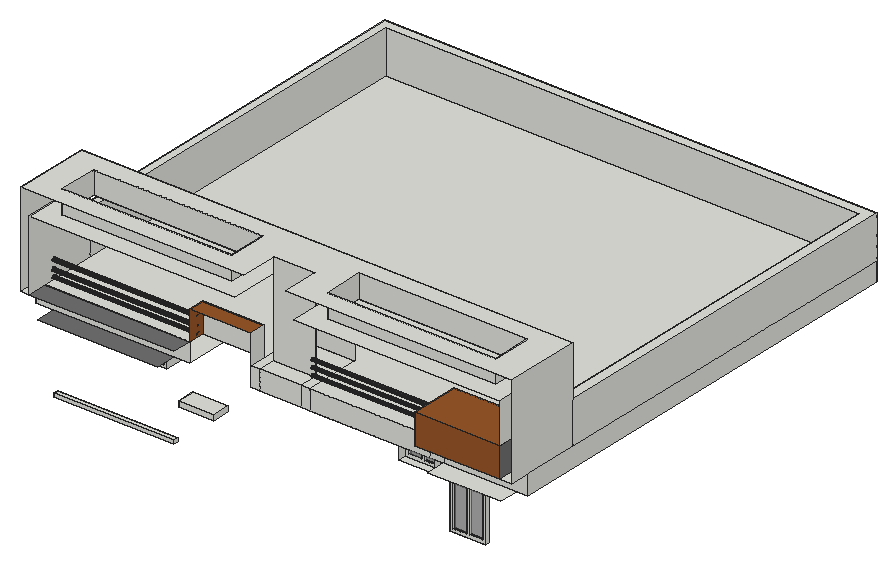
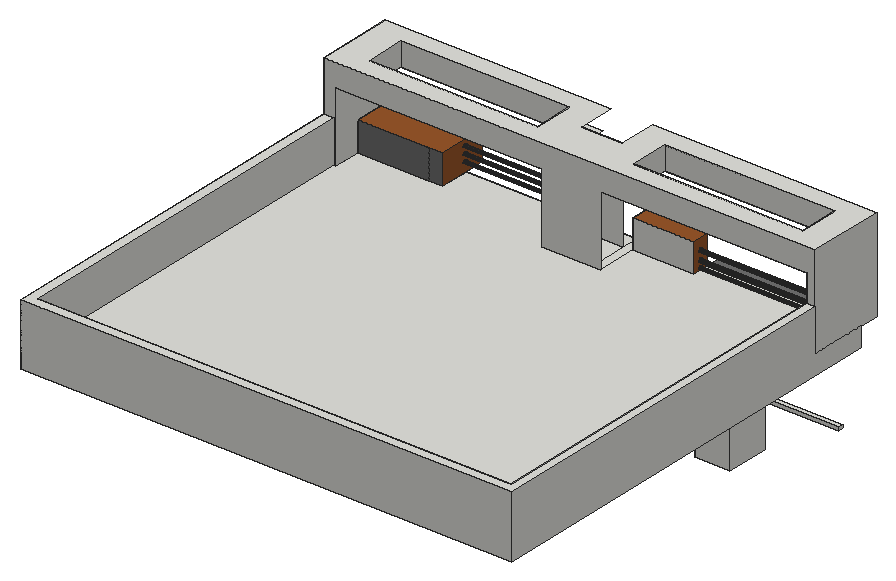
# SketchUp Ruby script. Lengths in inches.
U = 1.inch
M = Sketchup.active_model
def pt(a) = Geom::Point3d.new(a.map { |v| v * U })
def face(e, loops, mat)
  f = e.add_face(loops[0].map { |a| pt(a) })
  loops[1..].each { |l| e.add_face(l.map { |a| pt(a) }).erase! }
  f.material = f.back_material = mat if mat
  f
end
# faces: each face lists its corners as indices into pts; further lists are holes
def faces(e, pts, list, mat = nil) = list.each { |f| face(e, (f[0].is_a?(Array) ? f : [f]).map { |l| l.map { |i| pts[i] } }, mat) }
# xy, xz, yz: faces in a plane at the given z, y or x. An outline is a flat list of corners, or four numbers for a rectangle; further outlines are holes
def ring(l) = l.size == 4 ? [[l[0], l[1]], [l[2], l[1]], [l[2], l[3]], [l[0], l[3]]] : l.each_slice(2).to_a
def flat(e, list, mat, &to3) = list.each { |f| face(e, (f[0].is_a?(Array) ? f : [f]).map { |l| ring(l).map { |u, v| to3.(u, v) } }, mat) }
def xy(e, z, list, mat = nil) = flat(e, list, mat) { |x, y| [x, y, z] }
def xz(e, y, list, mat = nil) = flat(e, list, mat) { |x, z| [x, y, z] }
def yz(e, x, list, mat = nil) = flat(e, list, mat) { |y, z| [x, y, z] }
def lines(e, pts, list) = list.each { |a, b| e.add_line(pt(pts[a]), pt(pts[b])) }
# prism: a flat outline (further loops are holes) pulled along v
def prism(e, loops, v, mat = nil)
  f = face(e, loops, mat); d = Geom::Vector3d.new(v.map { |x| x * U })
  f.pushpull(f.normal.samedirection?(d) ? d.length : -d.length)
end
def box(e, o, s, mat = nil) = prism(e, [[o, [o[0] + s[0], o[1], o[2]], [o[0] + s[0], o[1] + s[1], o[2]], [o[0], o[1] + s[1], o[2]]]], [0, 0, s[2]], mat)
def at(x, y, z, deg = 0) = Geom::Transformation.translation(pt([x, y, z])) * Geom::Transformation.rotation(ORIGIN, Z_AXIS, deg.degrees)
def axes(o, x, y, z) = Geom::Transformation.new([*x, 0, *y, 0, *z, 0, *pt(o).to_a, 1])
def part(name) = M.definitions.add(name)
# library, detail: a bought-in or finely detailed component or shape, given as its bounding box
def library(name, o, s) = part(name).tap { |d| box(d.entities, o, s) }
def detail(e, o, s) = box(e.add_group.entities, o, s)
def put(e, d, t, mat = nil) = e.add_instance(d, t).tap { |i| i.material = mat if mat }
def group(e, t, mat = nil) = e.add_group.tap { |g| g.transformation = t; g.material = mat if mat }.entities
root = M.entities
M.materials.add("Generic").color = [112, 112, 112]
M.materials.add("[Color M07]").color = [58, 58, 58]
M.materials.add("[Translucent Glass Gray]").color = [128, 128, 128]
M.materials["[Translucent Glass Gray]"].alpha = 0.5
M.materials.add("[Wood Cherry Original]").color = [152, 86, 42]
c1 = part("Group\#2")
xy(c1.entities,0,[[0,0,49,5]])
xy(c1.entities,4.23,[[4.23,0,22.39,2],[26.61,0,44.77,2]])
xy(c1.entities,60.71,[[4.23,0,22.39,2],[26.61,0,44.77,2]])
xy(c1.entities,64.9375,[[0,0,49,5]])
xz(c1.entities,0,[[[0,0,49,64.9375],[26.61,4.23,44.77,60.71],[4.23,4.23,22.39,60.71]]])
xz(c1.entities,2,[[4.23,4.23,22.39,60.71],[26.61,4.23,44.77,60.71]],"[Translucent Glass Gray]")
xz(c1.entities,5,[[0,0,49,64.9375]],"[Translucent Glass Gray]")
yz(c1.entities,0,[[0,0,5,64.9375]])
yz(c1.entities,4.23,[[0,4.23,2,60.71]])
yz(c1.entities,22.39,[[0,4.23,2,60.71]])
yz(c1.entities,26.61,[[0,4.23,2,60.71]])
yz(c1.entities,44.77,[[0,4.23,2,60.71]])
yz(c1.entities,49,[[0,0,5,64.9375]])
box(root,[24,106.875,891],[165.05,7.3125,4.75])
xy(root,903.58,[[46.11,213.8125,95.11,273.4375],[414.49,213.8125,463.49,273.4375]])
xy(root,957.51,[[216.02,81.875,264.46,106.875]])
xy(root,964.95,[[216.02,81.875,264.46,106.875]])
xy(root,968.52,[[46.11,213.8125,95.11,273.4375],[414.49,213.8125,463.49,273.4375]])
xy(root,973,[[124.42,213.8125,178.54,273.4375],[492.79,213.8125,546.92,273.4375]])
xy(root,998.375,[[561.52,79.8125,661.8125,106.875],[24,106.875,211.17,213.8125],[295.66,106.875,295.66,249.5625,347.59,249.5625,347.59,151,307.66,151,307.66,106.875],[307.66,106.875,364.97,151],[364.97,106.875,364.97,151,347.59,151,347.59,249.5625,376.97,249.5625,376.97,106.875],
  [376.97,106.875,561.52,213.8125]])
xy(root,998.375,[[24,79.8125,189.05,106.875]],"Generic")
xy(root,1025.25,[[0,79.8125,12,106.875],[659.375,79.8125,676.6875,106.875],[0,106.875,12,184.9375],[12,106.875,211.17,106.875,211.17,129.125,295.66,129.125,295.66,184.9375,376.97,184.9375,376.97,106.875,542.64,106.875,542.64,147.5,659.375,147.5,659.375,184.9375,662.75,184.9375,662.75,693.375,12,693.375],[295.66,106.875,307.66,184.9375],
  [307.66,106.875,364.97,130.875],[364.97,106.875,376.97,106.875,376.97,184.9375,307.66,184.9375,307.66,130.875,364.97,130.875],[659.375,106.875,676.6875,184.9375]])
xy(root,1025.25,[[12,79.8125,211.17,106.875],[542.64,79.8125,659.375,106.875],[542.64,106.875,561.52,147.5],[561.52,106.875,659.375,147.5]],"Generic")
xy(root,1065.0625,[[211.17,106.875,295.66,129.125]],"[Wood Cherry Original]")
xy(root,1066.4375,[[542.64,79.8125,659.375,147.5]],"[Wood Cherry Original]")
xy(root,1084,[[0,184.9375,12,184.9375,12,693.375,662.75,693.375,662.75,184.9375,676.6875,184.9375,676.6875,706.875,0,706.875]])
xy(root,1121.625,[[[12,79.8125,295.66,184.9375],[37.42,105.23,270.24,159.52]],[[376.97,79.8125,659.375,184.9375],[402.39,105.23,633.96,159.52]]])
xy(root,1153.3125,[[[0,79.8125,307.66,79.8125,307.66,130.875,364.97,130.875,364.97,79.8125,676.6875,79.8125,676.6875,184.9375,0,184.9375],[37.42,105.23,270.24,159.52],[402.39,105.23,633.96,159.52]]])
xz(root,79.8125,[[542.64,1025.25,659.375,1066.4375]],"[Wood Cherry Original]")
xz(root,81.875,[[216.02,957.51,264.46,964.95]])
xz(root,105.23,[[37.42,1121.625,270.24,1153.3125],[402.39,1121.625,633.96,1153.3125]])
xz(root,106.875,[[0,998.375,211.17,1025.25],[295.66,998.375,307.66,1025.25],[307.66,998.375,364.97,1025.25],[364.97,998.375,376.97,1025.25],[376.97,998.375,542.64,1025.25],
  [542.64,998.375,561.52,1025.25],[561.52,998.375,676.6875,1025.25]])
xz(root,129.125,[[211.17,1025.25,295.66,1065.0625]])
xz(root,130.875,[[307.66,1025.25,364.97,1153.3125]])
xz(root,147.5,[[542.64,1025.25,561.52,1066.4375],[561.52,1025.25,659.375,1066.4375]],"Generic")
xz(root,159.52,[[37.42,1121.625,270.24,1153.3125],[402.39,1121.625,633.96,1153.3125]])
xz(root,184.9375,[[0,1025.25,12,1084],[295.66,1025.25,295.66,1121.625,12,1121.625,12,1084,0,1084,0,1153.3125,676.6875,1153.3125,676.6875,1084,662.75,1084,662.75,1071.0625,659.375,1071.0625,659.375,1121.625,376.97,1121.625,376.97,1025.25],[659.375,1025.25,662.75,1071.0625],[662.75,1025.25,676.6875,1084]])
xz(root,273.4375,[[46.11,903.58,95.11,968.52],[414.49,903.58,463.49,968.52]])
xz(root,693.375,[[12,1025.25,662.75,1084]])
xz(root,706.875,[[0,998.375,676.6875,1084]])
yz(root,0,[[106.875,998.375,106.875,1025.25,184.9375,1025.25,184.9375,1084,706.875,1084,706.875,998.375],[79.8125,1025.25,184.9375,1153.3125]])
yz(root,12,[[[79.8125,1025.25,184.9375,1121.625],[120.64,1049.14,120.125,1049.16,119.625,1049.31,119.18,1049.59,118.82,1049.97,118.58,1050.43,118.46,1050.94,118.48,1051.46,118.63,1051.96,118.9,1052.4,119.28,1052.76,119.75,1053,120.25,1053.12,120.78,1053.1,121.28,1052.95,121.72,1052.68,122.08,1052.3,122.32,1051.83,122.44,1051.33,122.42,1050.8,122.27,1050.3,122,1049.86,121.61,1049.5,121.15,1049.26],[120.45,1036.69,119.93,1036.76,119.45,1036.96,119.04,1037.28,118.72,1037.69,118.52,1038.18,118.45,1038.69,118.52,1039.21,118.72,1039.69,119.04,1040.11,119.45,1040.43,119.93,1040.625,120.45,1040.69,120.97,1040.625,121.45,1040.43,121.86,1040.11,122.18,1039.69,122.38,1039.21,122.45,1038.69,122.38,1038.18,122.18,1037.69,121.86,1037.28,121.45,1036.96,120.97,1036.76],[120.45,1027.44,119.93,1027.51,119.45,1027.71,119.04,1028.03,118.72,1028.44,118.52,1028.93,118.45,1029.44,118.52,1029.96,118.72,1030.44,119.04,1030.86,119.45,1031.18,119.93,1031.375,120.45,1031.44,120.97,1031.375,121.45,1031.18,121.86,1030.86,122.18,1030.44,122.38,1029.96,122.45,1029.44,122.38,1028.93,122.18,1028.44,121.86,1028.03,121.45,1027.71,120.97,1027.51]],[184.9375,1025.25,693.375,1084]])
yz(root,37.42,[[105.23,1121.625,159.52,1153.3125]])
yz(root,46.11,[[213.8125,903.58,273.4375,968.52]])
yz(root,95.11,[[213.8125,903.58,273.4375,968.52]])
yz(root,211.17,[[[106.875,1025.25,129.125,1065.0625],[120.64,1049.14,121.15,1049.26,121.61,1049.5,122,1049.86,122.27,1050.3,122.42,1050.8,122.44,1051.33,122.32,1051.83,122.08,1052.3,121.72,1052.68,121.28,1052.95,120.78,1053.1,120.25,1053.12,119.75,1053,119.28,1052.76,118.9,1052.4,118.63,1051.96,118.48,1051.46,118.46,1050.94,118.58,1050.43,118.82,1049.97,119.18,1049.59,119.625,1049.31,120.125,1049.16],[120.45,1027.44,120.97,1027.51,121.45,1027.71,121.86,1028.03,122.18,1028.44,122.38,1028.93,122.45,1029.44,122.38,1029.96,122.18,1030.44,121.86,1030.86,121.45,1031.18,120.97,1031.375,120.45,1031.44,119.93,1031.375,119.45,1031.18,119.04,1030.86,118.72,1030.44,118.52,1029.96,118.45,1029.44,118.52,1028.93,118.72,1028.44,119.04,1028.03,119.45,1027.71,119.93,1027.51],[120.45,1036.69,120.97,1036.76,121.45,1036.96,121.86,1037.28,122.18,1037.69,122.38,1038.18,122.45,1038.69,122.38,1039.21,122.18,1039.69,121.86,1040.11,121.45,1040.43,120.97,1040.625,120.45,1040.69,119.93,1040.625,119.45,1040.43,119.04,1040.11,118.72,1039.69,118.52,1039.21,118.45,1038.69,118.52,1038.18,118.72,1037.69,119.04,1037.28,119.45,1036.96,119.93,1036.76]],[120.45,1027.44,120.97,1027.51,121.45,1027.71,121.86,1028.03,122.18,1028.44,122.38,1028.93,122.45,1029.44,122.38,1029.96,122.18,1030.44,121.86,1030.86,121.45,1031.18,120.97,1031.375,120.45,1031.44,119.93,1031.375,119.45,1031.18,119.04,1030.86,118.72,1030.44,118.52,1029.96,118.45,1029.44,118.52,1028.93,118.72,1028.44,119.04,1028.03,119.45,1027.71,119.93,1027.51],[120.45,1036.69,120.97,1036.76,121.45,1036.96,121.86,1037.28,122.18,1037.69,122.38,1038.18,122.45,1038.69,122.38,1039.21,122.18,1039.69,121.86,1040.11,121.45,1040.43,120.97,1040.625,120.45,1040.69,119.93,1040.625,119.45,1040.43,119.04,1040.11,118.72,1039.69,118.52,1039.21,118.45,1038.69,118.52,1038.18,118.72,1037.69,119.04,1037.28,119.45,1036.96,119.93,1036.76],[120.64,1049.14,121.15,1049.26,121.61,1049.5,122,1049.86,122.27,1050.3,122.42,1050.8,122.44,1051.33,122.32,1051.83,122.08,1052.3,121.72,1052.68,121.28,1052.95,120.78,1053.1,120.25,1053.12,119.75,1053,119.28,1052.76,118.9,1052.4,118.63,1051.96,118.48,1051.46,118.46,1050.94,118.58,1050.43,118.82,1049.97,119.18,1049.59,119.625,1049.31,120.125,1049.16]],"[Wood Cherry Original]")
yz(root,216.02,[[81.875,957.51,106.875,964.95]])
yz(root,264.46,[[81.875,957.51,106.875,964.95]])
yz(root,270.24,[[105.23,1121.625,159.52,1153.3125]])
yz(root,295.66,[[106.875,1025.25,129.125,1065.0625]])
yz(root,402.39,[[105.23,1121.625,159.52,1153.3125]])
yz(root,414.49,[[213.8125,903.58,273.4375,968.52]])
yz(root,463.49,[[213.8125,903.58,273.4375,968.52]])
yz(root,542.64,[[[79.8125,1025.25,147.5,1066.4375],[111.28,1047.72,111.79,1047.78,112.28,1047.98,112.69,1048.3,113.01,1048.72,113.21,1049.2,113.28,1049.72,113.21,1050.23,113.01,1050.72,112.69,1051.13,112.28,1051.45,111.79,1051.65,111.28,1051.72,110.76,1051.65,110.28,1051.45,109.86,1051.13,109.55,1050.72,109.35,1050.23,109.28,1049.72,109.35,1049.2,109.55,1048.72,109.86,1048.3,110.28,1047.98,110.76,1047.78],[111.28,1038.03,111.79,1038.1,112.28,1038.3,112.69,1038.61,113.01,1039.03,113.21,1039.51,113.28,1040.03,113.21,1040.55,113.01,1041.03,112.69,1041.44,112.28,1041.76,111.79,1041.96,111.28,1042.03,110.76,1041.96,110.28,1041.76,109.86,1041.44,109.55,1041.03,109.35,1040.55,109.28,1040.03,109.35,1039.51,109.55,1039.03,109.86,1038.61,110.28,1038.3,110.76,1038.1],[111.28,1057.4,111.79,1057.47,112.28,1057.67,112.69,1057.99,113.01,1058.4,113.21,1058.89,113.28,1059.4,113.21,1059.92,113.01,1060.4,112.69,1060.82,112.28,1061.14,111.79,1061.34,111.28,1061.4,110.76,1061.34,110.28,1061.14,109.86,1060.82,109.55,1060.4,109.35,1059.92,109.28,1059.4,109.35,1058.89,109.55,1058.4,109.86,1057.99,110.28,1057.67,110.76,1057.47]],[111.28,1038.03,111.79,1038.1,112.28,1038.3,112.69,1038.61,113.01,1039.03,113.21,1039.51,113.28,1040.03,113.21,1040.55,113.01,1041.03,112.69,1041.44,112.28,1041.76,111.79,1041.96,111.28,1042.03,110.76,1041.96,110.28,1041.76,109.86,1041.44,109.55,1041.03,109.35,1040.55,109.28,1040.03,109.35,1039.51,109.55,1039.03,109.86,1038.61,110.28,1038.3,110.76,1038.1],[111.28,1047.72,111.79,1047.78,112.28,1047.98,112.69,1048.3,113.01,1048.72,113.21,1049.2,113.28,1049.72,113.21,1050.23,113.01,1050.72,112.69,1051.13,112.28,1051.45,111.79,1051.65,111.28,1051.72,110.76,1051.65,110.28,1051.45,109.86,1051.13,109.55,1050.72,109.35,1050.23,109.28,1049.72,109.35,1049.2,109.55,1048.72,109.86,1048.3,110.28,1047.98,110.76,1047.78],[111.28,1057.4,111.79,1057.47,112.28,1057.67,112.69,1057.99,113.01,1058.4,113.21,1058.89,113.28,1059.4,113.21,1059.92,113.01,1060.4,112.69,1060.82,112.28,1061.14,111.79,1061.34,111.28,1061.4,110.76,1061.34,110.28,1061.14,109.86,1060.82,109.55,1060.4,109.35,1059.92,109.28,1059.4,109.35,1058.89,109.55,1058.4,109.86,1057.99,110.28,1057.67,110.76,1057.47]],"[Wood Cherry Original]")
yz(root,633.96,[[105.23,1121.625,159.52,1153.3125]])
yz(root,659.375,[[147.5,1025.25,147.5,1066.4375,79.8125,1066.4375,79.8125,1121.625,184.9375,1121.625,184.9375,1025.25]])
yz(root,659.375,[[79.8125,1025.25,147.5,1066.4375]],"Generic")
yz(root,662.75,[[184.9375,1025.25,693.375,1084]])
yz(root,676.6875,[[106.875,998.375,706.875,1025.25],[79.8125,1025.25,184.9375,1153.3125],[184.9375,1025.25,706.875,1084]])
p = [[211.17,120.45,1027.44],[211.17,119.93,1027.51],[12,119.93,1027.51],[12,120.45,1027.44],[211.17,120.97,1027.51],[12,120.97,1027.51],
  [211.17,119.45,1027.71],[12,119.45,1027.71],[211.17,121.45,1027.71],[12,121.45,1027.71],[211.17,119.04,1028.03],[12,119.04,1028.03],
  [211.17,121.86,1028.03],[12,121.86,1028.03],[211.17,118.72,1028.44],[12,118.72,1028.44],[211.17,122.18,1028.44],[12,122.18,1028.44],
  [211.17,118.52,1028.93],[12,118.52,1028.93],[211.17,122.38,1028.93],[12,122.38,1028.93],[211.17,118.45,1029.44],[12,118.45,1029.44],
  [211.17,122.45,1029.44],[12,122.45,1029.44],[211.17,118.52,1029.96],[12,118.52,1029.96],[211.17,122.38,1029.96],[12,122.38,1029.96],
  [211.17,118.72,1030.44],[12,118.72,1030.44],[211.17,122.18,1030.44],[12,122.18,1030.44],[211.17,119.04,1030.86],[12,119.04,1030.86],
  [211.17,121.86,1030.86],[12,121.86,1030.86],[211.17,119.45,1031.18],[12,119.45,1031.18],[211.17,121.45,1031.18],[12,121.45,1031.18],
  [211.17,119.93,1031.375],[12,119.93,1031.375],[211.17,120.97,1031.375],[12,120.97,1031.375],[211.17,120.45,1031.44],[12,120.45,1031.44],
  [211.17,120.45,1036.69],[211.17,119.93,1036.76],[12,119.93,1036.76],[12,120.45,1036.69],[211.17,120.97,1036.76],[12,120.97,1036.76],
  [211.17,119.45,1036.96],[12,119.45,1036.96],[211.17,121.45,1036.96],[12,121.45,1036.96],[211.17,119.04,1037.28],[12,119.04,1037.28],
  [211.17,121.86,1037.28],[12,121.86,1037.28],[211.17,118.72,1037.69],[12,118.72,1037.69],[211.17,122.18,1037.69],[12,122.18,1037.69],
  [211.17,118.52,1038.18],[12,118.52,1038.18],[211.17,122.38,1038.18],[12,122.38,1038.18],[542.64,111.28,1038.03],[542.64,110.76,1038.1],
  [376.97,110.76,1038.1],[376.97,111.28,1038.03],[542.64,111.79,1038.1],[376.97,111.79,1038.1],[542.64,110.28,1038.3],[376.97,110.28,1038.3],
  [542.64,112.28,1038.3],[376.97,112.28,1038.3],[211.17,118.45,1038.69],[12,118.45,1038.69],[211.17,122.45,1038.69],[12,122.45,1038.69],
  [542.64,109.86,1038.61],[376.97,109.86,1038.61],[542.64,112.69,1038.61],[376.97,112.69,1038.61],[542.64,109.55,1039.03],[376.97,109.55,1039.03],
  [542.64,113.01,1039.03],[376.97,113.01,1039.03],[211.17,118.52,1039.21],[12,118.52,1039.21],[211.17,122.38,1039.21],[12,122.38,1039.21],
  [542.64,109.35,1039.51],[376.97,109.35,1039.51],[542.64,113.21,1039.51],[376.97,113.21,1039.51],[211.17,118.72,1039.69],[12,118.72,1039.69],
  [211.17,122.18,1039.69],[12,122.18,1039.69],[542.64,109.28,1040.03],[376.97,109.28,1040.03],[542.64,113.28,1040.03],[376.97,113.28,1040.03],
  [211.17,119.04,1040.11],[12,119.04,1040.11],[211.17,121.86,1040.11],[12,121.86,1040.11],[542.64,109.35,1040.55],[376.97,109.35,1040.55],
  [542.64,113.21,1040.55],[376.97,113.21,1040.55],[211.17,119.45,1040.43],[12,119.45,1040.43],[211.17,121.45,1040.43],[12,121.45,1040.43],
  [211.17,119.93,1040.625],[12,119.93,1040.625],[211.17,120.97,1040.625],[12,120.97,1040.625],[542.64,109.55,1041.03],[376.97,109.55,1041.03],
  [542.64,113.01,1041.03],[376.97,113.01,1041.03],[211.17,120.45,1040.69],[12,120.45,1040.69],[542.64,109.86,1041.44],[376.97,109.86,1041.44],
  [542.64,112.69,1041.44],[376.97,112.69,1041.44],[542.64,110.28,1041.76],[376.97,110.28,1041.76],[542.64,112.28,1041.76],[376.97,112.28,1041.76],
  [542.64,110.76,1041.96],[376.97,110.76,1041.96],[542.64,111.79,1041.96],[376.97,111.79,1041.96],[542.64,111.28,1042.03],[376.97,111.28,1042.03],
  [542.64,111.28,1047.72],[542.64,110.76,1047.78],[376.97,110.76,1047.78],[376.97,111.28,1047.72],[542.64,111.79,1047.78],[376.97,111.79,1047.78],
  [542.64,110.28,1047.98],[376.97,110.28,1047.98],[542.64,112.28,1047.98],[376.97,112.28,1047.98],[542.64,109.86,1048.3],[376.97,109.86,1048.3],
  [542.64,112.69,1048.3],[376.97,112.69,1048.3],[542.64,109.55,1048.72],[376.97,109.55,1048.72],[542.64,113.01,1048.72],[376.97,113.01,1048.72],
  [542.64,109.35,1049.2],[376.97,109.35,1049.2],[542.64,113.21,1049.2],[376.97,113.21,1049.2],[211.17,120.64,1049.14],[211.17,120.125,1049.16],
  [12,120.125,1049.16],[12,120.64,1049.14],[211.17,121.15,1049.26],[12,121.15,1049.26],[542.64,109.28,1049.72],[376.97,109.28,1049.72],
  [542.64,113.28,1049.72],[376.97,113.28,1049.72],[211.17,119.625,1049.31],[12,119.625,1049.31],[211.17,119.18,1049.59],[12,119.18,1049.59],
  [211.17,121.61,1049.5],[12,121.61,1049.5],[211.17,122,1049.86],[12,122,1049.86],[211.17,118.82,1049.97],[12,118.82,1049.97],
  [542.64,109.35,1050.23],[376.97,109.35,1050.23],[542.64,113.21,1050.23],[376.97,113.21,1050.23],[211.17,122.27,1050.3],[12,122.27,1050.3],
  [211.17,118.58,1050.43],[12,118.58,1050.43],[542.64,109.55,1050.72],[376.97,109.55,1050.72],[542.64,113.01,1050.72],[376.97,113.01,1050.72],
  [211.17,122.42,1050.8],[12,122.42,1050.8],[211.17,118.46,1050.94],[12,118.46,1050.94],[542.64,109.86,1051.13],[376.97,109.86,1051.13],
  [542.64,112.69,1051.13],[376.97,112.69,1051.13],[211.17,122.44,1051.33],[12,122.44,1051.33],[211.17,118.48,1051.46],[12,118.48,1051.46],
  [542.64,110.28,1051.45],[376.97,110.28,1051.45],[542.64,112.28,1051.45],[376.97,112.28,1051.45],[211.17,122.32,1051.83],[12,122.32,1051.83],
  [542.64,110.76,1051.65],[376.97,110.76,1051.65],[542.64,111.79,1051.65],[376.97,111.79,1051.65],[211.17,118.63,1051.96],[12,118.63,1051.96],
  [542.64,111.28,1051.72],[376.97,111.28,1051.72],[211.17,122.08,1052.3],[12,122.08,1052.3],[211.17,118.9,1052.4],[12,118.9,1052.4],
  [211.17,121.72,1052.68],[12,121.72,1052.68],[211.17,119.28,1052.76],[12,119.28,1052.76],[211.17,121.28,1052.95],[12,121.28,1052.95],
  [211.17,119.75,1053],[12,119.75,1053],[211.17,120.25,1053.12],[12,120.25,1053.12],[211.17,120.78,1053.1],[12,120.78,1053.1],
  [542.64,111.28,1057.4],[542.64,110.76,1057.47],[376.97,110.76,1057.47],[376.97,111.28,1057.4],[542.64,111.79,1057.47],[376.97,111.79,1057.47],
  [542.64,110.28,1057.67],[376.97,110.28,1057.67],[542.64,112.28,1057.67],[376.97,112.28,1057.67],[542.64,109.86,1057.99],[376.97,109.86,1057.99],
  [542.64,112.69,1057.99],[376.97,112.69,1057.99],[542.64,109.55,1058.4],[376.97,109.55,1058.4],[542.64,113.01,1058.4],[376.97,113.01,1058.4],
  [542.64,109.35,1058.89],[376.97,109.35,1058.89],[542.64,113.21,1058.89],[376.97,113.21,1058.89],[542.64,109.28,1059.4],[376.97,109.28,1059.4],
  [542.64,113.28,1059.4],[376.97,113.28,1059.4],[542.64,109.35,1059.92],[376.97,109.35,1059.92],[542.64,113.21,1059.92],[376.97,113.21,1059.92],
  [542.64,109.55,1060.4],[376.97,109.55,1060.4],[542.64,113.01,1060.4],[376.97,113.01,1060.4],[542.64,109.86,1060.82],[376.97,109.86,1060.82],
  [542.64,112.69,1060.82],[376.97,112.69,1060.82],[542.64,110.28,1061.14],[376.97,110.28,1061.14],[542.64,112.28,1061.14],[376.97,112.28,1061.14],
  [542.64,110.76,1061.34],[376.97,110.76,1061.34],[542.64,111.79,1061.34],[376.97,111.79,1061.34],[542.64,111.28,1061.4],[376.97,111.28,1061.4],
  [368.81,128.38,1025.25],[368.81,128.38,1116.625],[211.17,120.45,1038.69],[12,120.45,1038.69],[211.17,120.45,1051.13],[12,120.45,1051.13],
  [211.17,120.45,1029.44],[12,120.45,1029.44],[542.64,111.28,1040.03],[376.97,111.28,1040.03],[542.64,111.28,1049.72],[376.97,111.28,1049.72],
  [542.64,111.28,1059.4],[376.97,111.28,1059.4]]
faces(root,p,[[0,1,2,3],[4,0,3,5],[1,6,7,2],[8,4,5,9],[6,10,11,7],[12,8,9,13],[10,14,15,11],[16,12,13,17],
  [14,18,19,15],[20,16,17,21],[18,22,23,19],[24,20,21,25],[22,26,27,23],[28,24,25,29],[26,30,31,27],[32,28,29,33],
  [30,34,35,31],[36,32,33,37],[34,38,39,35],[40,36,37,41],[38,42,43,39],[44,40,41,45],[42,46,47,43],[46,44,45,47],
  [48,49,50,51],[52,48,51,53],[49,54,55,50],[56,52,53,57],[54,58,59,55],[60,56,57,61],[58,62,63,59],[64,60,61,65],
  [62,66,67,63],[68,64,65,69],[70,71,72,73],[74,70,73,75],[71,76,77,72],[78,74,75,79],[66,80,81,67],[82,68,69,83],
  [76,84,85,77],[86,78,79,87],[84,88,89,85],[90,86,87,91],[80,92,93,81],[94,82,83,95],[88,96,97,89],[98,90,91,99],
  [92,100,101,93],[102,94,95,103],[96,104,105,97],[106,98,99,107],[100,108,109,101],[110,102,103,111],[104,112,113,105],[114,106,107,115],
  [108,116,117,109],[118,110,111,119],[116,120,121,117],[122,118,119,123],[112,124,125,113],[126,114,115,127],[120,128,129,121],[128,122,123,129],
  [124,130,131,125],[132,126,127,133],[130,134,135,131],[136,132,133,137],[134,138,139,135],[140,136,137,141],[138,142,143,139],[142,140,141,143],
  [144,145,146,147],[148,144,147,149],[145,150,151,146],[152,148,149,153],[150,154,155,151],[156,152,153,157],[154,158,159,155],[160,156,157,161],
  [158,162,163,159],[164,160,161,165],[166,167,168,169],[170,166,169,171],[162,172,173,163],[174,164,165,175],[167,176,177,168],[176,178,179,177],
  [180,170,171,181],[182,180,181,183],[178,184,185,179],[172,186,187,173],[188,174,175,189],[190,182,183,191],[184,192,193,185],[186,194,195,187],
  [196,188,189,197],[198,190,191,199],[192,200,201,193],[194,202,203,195],[204,196,197,205],[206,198,199,207],[200,208,209,201],[202,210,211,203],
  [212,204,205,213],[214,206,207,215],[210,216,217,211],[218,212,213,219],[208,220,221,209],[216,222,223,217],[222,218,219,223],[224,214,215,225],
  [220,226,227,221],[228,224,225,229],[226,230,231,227],[232,228,229,233],[230,234,235,231],[234,236,237,235],[238,232,233,239],[236,238,239,237],
  [240,241,242,243],[244,240,243,245],[241,246,247,242],[248,244,245,249],[246,250,251,247],[252,248,249,253],[250,254,255,251],[256,252,253,257],
  [254,258,259,255],[260,256,257,261],[258,262,263,259],[264,260,261,265],[262,266,267,263],[268,264,265,269],[266,270,271,267],[272,268,269,273],
  [270,274,275,271],[276,272,273,277],[274,278,279,275],[280,276,277,281],[278,282,283,279],[284,280,281,285],[282,286,287,283],[286,284,285,287]],"[Color M07]")
lines(root,p,[[288,289],[290,291],[292,293],[294,295],[296,297],[298,299],[300,301]])
put(root,c1,at(414.49,224.0625,903.58))
put(root,c1,at(46.11,213.8125,903.58))
put(root,c1,at(573.95,101.875,921.54))
